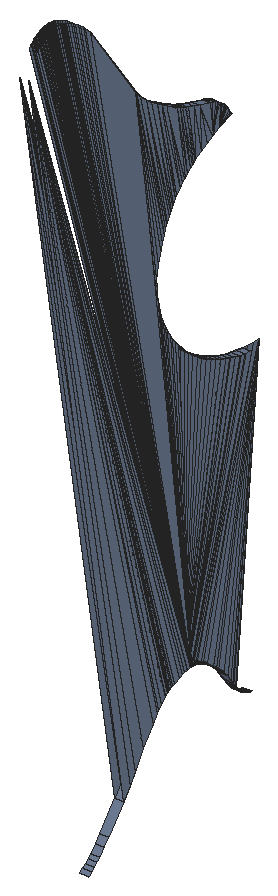
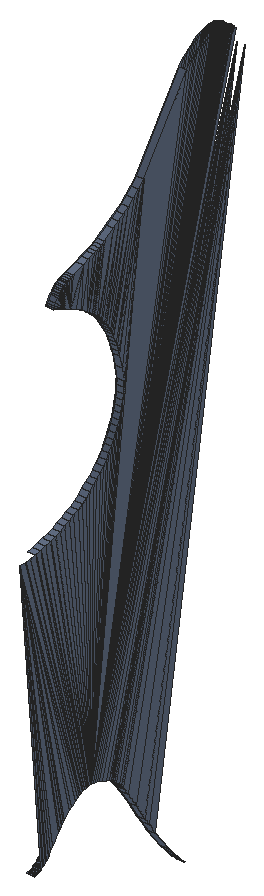
# SketchUp Ruby script. Lengths in inches.
U = 1.inch
M = Sketchup.active_model
def pt(a) = Geom::Point3d.new(a.map { |v| v * U })
def face(e, loops, mat)
  f = e.add_face(loops[0].map { |a| pt(a) })
  loops[1..].each { |l| e.add_face(l.map { |a| pt(a) }).erase! }
  f.material = f.back_material = mat if mat
  f
end
# faces: each face lists its corners as indices into pts; further lists are holes
def faces(e, pts, list, mat = nil) = list.each { |f| face(e, (f[0].is_a?(Array) ? f : [f]).map { |l| l.map { |i| pts[i] } }, mat) }
# xy, xz, yz: faces in a plane at the given z, y or x. An outline is a flat list of corners, or four numbers for a rectangle; further outlines are holes
def ring(l) = l.size == 4 ? [[l[0], l[1]], [l[2], l[1]], [l[2], l[3]], [l[0], l[3]]] : l.each_slice(2).to_a
def flat(e, list, mat, &to3) = list.each { |f| face(e, (f[0].is_a?(Array) ? f : [f]).map { |l| ring(l).map { |u, v| to3.(u, v) } }, mat) }
def xy(e, z, list, mat = nil) = flat(e, list, mat) { |x, y| [x, y, z] }
def xz(e, y, list, mat = nil) = flat(e, list, mat) { |x, z| [x, y, z] }
def yz(e, x, list, mat = nil) = flat(e, list, mat) { |y, z| [x, y, z] }
def lines(e, pts, list) = list.each { |a, b| e.add_line(pt(pts[a]), pt(pts[b])) }
# prism: a flat outline (further loops are holes) pulled along v
def prism(e, loops, v, mat = nil)
  f = face(e, loops, mat); d = Geom::Vector3d.new(v.map { |x| x * U })
  f.pushpull(f.normal.samedirection?(d) ? d.length : -d.length)
end
def box(e, o, s, mat = nil) = prism(e, [[o, [o[0] + s[0], o[1], o[2]], [o[0] + s[0], o[1] + s[1], o[2]], [o[0], o[1] + s[1], o[2]]]], [0, 0, s[2]], mat)
def at(x, y, z, deg = 0) = Geom::Transformation.translation(pt([x, y, z])) * Geom::Transformation.rotation(ORIGIN, Z_AXIS, deg.degrees)
def axes(o, x, y, z) = Geom::Transformation.new([*x, 0, *y, 0, *z, 0, *pt(o).to_a, 1])
def part(name) = M.definitions.add(name)
# library, detail: a bought-in or finely detailed component or shape, given as its bounding box
def library(name, o, s) = part(name).tap { |d| box(d.entities, o, s) }
def detail(e, o, s) = box(e.add_group.entities, o, s)
def put(e, d, t, mat = nil) = e.add_instance(d, t).tap { |i| i.material = mat if mat }
def group(e, t, mat = nil) = e.add_group.tap { |g| g.transformation = t; g.material = mat if mat }.entities
root = M.entities
M.materials.add("3D66_SU_1584934530605_002").color = [112, 126, 151]
xy(root,58.92,[[122.5,258.88,123.07,258.94]],"3D66_SU_1584934530605_002")
xy(root,58.93,[[122.5,258.6875,123.07,258.75],[122.5,258.75,123.07,258.8125]],"3D66_SU_1584934530605_002")
yz(root,122.5,[[252.91,53.28,244.87,100.53,253.42,53.97],[253.42,53.97,244.87,100.53,253.83,54.59],[253.83,54.59,244.87,100.53,254.58,55.75],[263.16,55.41,263.09,55.45,265.06,75.81],[263.09,55.45,263.01,55.5,265.06,75.81],
  [263.01,55.5,262.94,55.55,265.06,75.81],[262.94,55.55,262.87,55.61,265.06,75.81],[262.87,55.61,262.8,55.66,265.06,75.81],[262.8,55.66,262.73,55.73,265.06,75.81],[262.73,55.73,262.6,55.86,265.06,75.81],
  [254.58,55.75,244.87,100.53,255.36,56.85],[262.6,55.86,262.47,56,265.06,75.81],[262.47,56,262.35,56.15,265.06,75.81],[262.35,56.15,262.11,56.47,265.06,75.81],[262.11,56.47,261.65,57.11,265.06,75.81],
  [255.36,56.85,244.87,100.53,255.74,57.33],[261.65,57.11,261.53,57.26,265.06,75.81],[261.53,57.26,261.41,57.4,265.06,75.81],[255.74,57.33,244.87,100.53,255.92,57.55],[261.41,57.4,261.29,57.52,265.06,75.81],
  [261.29,57.52,261.23,57.58,265.06,75.81],[255.92,57.55,244.87,100.53,256.09,57.74],[261.23,57.58,261.17,57.64,265.06,75.81],[261.17,57.64,260.66,58.06,265.06,75.81],[256.09,57.74,244.87,100.53,256.38,58.03],
  [256.38,58.03,244.87,100.53,256.51,58.14],[260.66,58.06,260.4,58.25,265.06,75.81],[256.51,58.14,244.87,100.53,256.57,58.19],[256.57,58.19,244.87,100.53,256.63,58.24],[256.63,58.24,244.87,100.53,256.7,58.28],
  [260.4,58.25,260.14,58.42,265.06,75.81],[256.7,58.28,244.87,100.53,256.76,58.32],[256.76,58.32,244.87,100.53,256.83,58.36],[256.83,58.36,244.87,100.53,256.9,58.4],[256.9,58.4,244.87,100.53,257.05,58.47],
  [260.14,58.42,259.88,58.58,265.06,75.81],[257.05,58.47,244.87,100.53,257.23,58.54],[257.23,58.54,244.87,100.53,257.65,58.7],[259.88,58.58,259.76,58.65,265.06,75.81],[259.76,58.65,259.63,58.71,265.06,75.81],
  [257.65,58.7,244.87,100.53,257.88,58.77],[259.63,58.71,259.5,58.77,264.58,75.82],[259.63,58.71,264.58,75.82,265.06,75.81],[257.88,58.77,244.87,100.53,258.12,58.84],[259.5,58.77,259.375,58.8125,264.58,75.82],
  [259.375,58.8125,259.25,58.85,264.1,75.85],[259.375,58.8125,264.1,75.85,264.58,75.82],[258.12,58.84,244.87,100.53,258.25,58.87],[259.25,58.85,259.1875,58.87,263.63,75.9],[259.25,58.85,263.63,75.9,264.1,75.85],
  [258.25,58.87,244.87,100.53,258.37,58.89],[259.1875,58.87,259.125,58.89,263.63,75.9],[258.37,58.89,244.87,100.53,258.5,58.91],[259.125,58.89,259.07,58.9,263.17,75.97],[259.125,58.89,263.17,75.97,263.63,75.9],
  [259.07,58.9,259,58.91,263.17,75.97],[258.5,58.91,244.87,100.53,258.625,58.92],[259,58.91,258.94,58.92,262.72,76.05],[259,58.91,262.72,76.05,263.17,75.97],[258.625,58.92,245.66,101.97,245.79,102.11],
  [258.625,58.92,245.79,102.11,245.85,102.18],[258.625,58.92,245.85,102.18,245.92,102.24],[258.625,58.92,245.92,102.24,245.99,102.3],[258.625,58.92,245.99,102.3,246.06,102.36],[258.625,58.92,246.06,102.36,246.13,102.41],
  [258.625,58.92,246.13,102.41,246.2,102.46],[258.625,58.92,246.2,102.46,246.27,102.51],[258.625,58.92,246.27,102.51,246.35,102.55],[258.625,58.92,246.35,102.55,246.42,102.59],[258.625,58.92,246.42,102.59,246.5,102.625],
  [258.625,58.92,246.5,102.625,246.57,102.65],[258.625,58.92,246.57,102.65,246.65,102.68],[258.625,58.92,246.65,102.68,246.73,102.7],[258.625,58.92,246.73,102.7,246.81,102.72],[258.625,58.92,246.81,102.72,246.89,102.74],
  [258.625,58.92,246.89,102.74,246.97,102.75],[258.625,58.92,246.97,102.75,247.05,102.76],[258.625,58.92,247.05,102.76,247.13,102.77],[258.625,58.92,247.13,102.77,247.22,102.77],[258.625,58.92,247.22,102.77,247.31,102.77],
  [258.625,58.92,247.31,102.77,247.39,102.76],[258.625,58.92,247.39,102.76,247.48,102.75],[258.625,58.92,247.48,102.75,247.57,102.74],[258.625,58.92,247.57,102.74,247.66,102.72],[258.625,58.92,247.66,102.72,247.75,102.7],
  [258.625,58.92,247.75,102.7,247.85,102.68],[258.625,58.92,247.85,102.68,247.94,102.65],[258.625,58.92,247.94,102.65,248.04,102.62],[258.625,58.92,248.04,102.62,248.23,102.54],[258.625,58.92,248.23,102.54,248.43,102.46],
  [258.625,58.92,248.43,102.46,248.625,102.35],[258.625,58.92,248.625,102.35,248.83,102.23],[258.625,58.92,248.83,102.23,249.03,102.1],[258.625,58.92,249.03,102.1,249.24,101.95],[258.625,58.92,249.24,101.95,249.45,101.79],
  [258.625,58.92,249.45,101.79,249.67,101.61],[258.625,58.92,249.67,101.61,250.1,101.21],[258.625,58.92,250.1,101.21,253.92,95.88],[258.625,58.92,253.92,95.88,255.73,82.82],[258.625,58.92,255.73,82.82,255.79,82.43],
  [258.625,58.92,255.79,82.43,255.875,82.05],[258.625,58.92,255.875,82.05,255.98,81.67],[258.625,58.92,255.98,81.67,256.11,81.3],[258.625,58.92,256.11,81.3,256.25,80.9375],[258.625,58.92,256.25,80.9375,256.42,80.58],
  [258.625,58.92,256.42,80.58,256.61,80.24],[258.625,58.92,256.61,80.24,256.82,79.9],[258.625,58.92,256.82,79.9,257.04,79.57],[258.625,58.92,257.04,79.57,257.29,79.25],[258.625,58.92,257.29,79.25,257.55,78.95],
  [258.625,58.92,257.55,78.95,257.83,78.65],[258.625,58.92,257.83,78.65,258.12,78.37],[258.625,58.92,258.12,78.37,258.43,78.1],[258.625,58.92,258.43,78.1,258.76,77.84],[258.625,58.92,258.76,77.84,259.1,77.59],
  [258.625,58.92,259.1,77.59,259.45,77.36],[258.625,58.92,259.45,77.36,259.82,77.14],[258.625,58.92,259.82,77.14,260.2,76.94],[258.625,58.92,260.2,76.94,260.59,76.75],[258.625,58.92,260.59,76.75,261,76.58],
  [258.625,58.92,261,76.58,261.41,76.42],[258.625,58.92,261.41,76.42,261.84,76.28],[258.625,58.92,261.84,76.28,258.6875,58.93],[258.88,58.92,258.8125,58.93,262.27,76.16],[258.88,58.92,262.27,76.16,262.72,76.05],
  [258.88,58.92,262.72,76.05,258.94,58.92],[258.6875,58.93,261.84,76.28,258.75,58.93],[258.75,58.93,261.84,76.28,262.27,76.16],[258.75,58.93,262.27,76.16,258.8125,58.93],[255.73,82.82,253.92,95.88,255.7,83.22],
  [255.7,83.22,253.92,95.88,255.68,83.62],[255.68,83.62,253.92,95.88,255.85,84.54],[255.85,84.54,253.92,95.88,256.05,85.37],[256.05,85.37,253.92,95.88,256.17,85.75],[256.17,85.75,253.92,95.88,256.3,86.12],
  [256.3,86.12,253.92,95.88,254.38,95.42],[256.3,86.12,254.38,95.42,256.44,86.46],[256.44,86.46,254.38,95.42,256.59,86.79],[256.59,86.79,254.38,95.42,254.83,95.03],[256.59,86.79,254.83,95.03,256.75,87.1],
  [256.75,87.1,254.83,95.03,256.92,87.39],[256.92,87.39,254.83,95.03,255.28,94.68],[256.92,87.39,255.28,94.68,257.1,87.66],[257.1,87.66,255.28,94.68,255.72,94.38],[257.1,87.66,255.72,94.38,257.28,87.92],
  [257.28,87.92,255.72,94.38,256.16,94.11],[257.28,87.92,256.16,94.11,257.47,88.17],[257.47,88.17,256.16,94.11,257.67,88.4],[257.67,88.4,256.16,94.11,256.6,93.86],[257.67,88.4,256.6,93.86,257.875,88.62],
  [257.875,88.62,256.6,93.86,258.09,88.82],[258.09,88.82,256.6,93.86,257.47,93.4],[258.09,88.82,257.47,93.4,258.31,89.02],[258.31,89.02,257.47,93.4,257.7,93.29],[258.31,89.02,257.7,93.29,258.53,89.2],
  [258.53,89.2,257.7,93.29,257.93,93.19],[258.53,89.2,257.93,93.19,258.76,89.375],[258.76,89.375,257.93,93.19,258.16,93.09],[258.76,89.375,258.16,93.09,258.99,89.54],[258.99,89.54,258.16,93.09,258.4,93.01],
  [258.99,89.54,258.4,93.01,258.88,92.86],[258.99,89.54,258.88,92.86,259.48,89.84],[259.48,89.84,258.88,92.86,259.35,92.72],[259.48,89.84,259.35,92.72,259.97,90.11],[259.97,90.11,259.35,92.72,260.48,90.36],
  [260.48,90.36,259.35,92.72,260.23,92.47],[260.48,90.36,260.23,92.47,260.43,92.41],[260.48,90.36,260.43,92.41,260.61,92.35],[260.48,90.36,260.61,92.35,260.78,92.28],[260.48,90.36,260.78,92.28,260.86,92.24],
  [260.48,90.36,260.86,92.24,260.93,92.21],[260.48,90.36,260.93,92.21,261.0625,92.13],[260.48,90.36,261.0625,92.13,261,90.59],[261,90.59,261.0625,92.13,261.18,92.06],[261,90.59,261.18,92.06,261.28,91.98],
  [261,90.59,261.28,91.98,261.375,91.91],[261,90.59,261.375,91.91,261.45,91.84],[261,90.59,261.45,91.84,261.52,91.76],[261,90.59,261.52,91.76,261.58,91.6875],[261,90.59,261.58,91.6875,261.64,91.61],
  [261,90.59,261.64,91.61,261.83,91.32],[261,90.59,261.83,91.32,261.93,91.17],[261,90.59,261.93,91.17,261.99,91.09],[261,90.59,261.99,91.09,262.06,91.02]],"3D66_SU_1584934530605_002")
yz(root,123.07,[[252.91,53.28,253.42,53.97,244.87,100.53],[253.42,53.97,253.83,54.59,244.87,100.53],[253.83,54.59,254.58,55.75,244.87,100.53],[254.58,55.75,255.36,56.85,244.87,100.53],[255.36,56.85,255.74,57.33,244.87,100.53],
  [255.74,57.33,255.92,57.55,244.87,100.53],[255.92,57.55,256.09,57.74,244.87,100.53],[256.09,57.74,256.38,58.03,244.87,100.53],[256.38,58.03,256.51,58.14,244.87,100.53],[256.51,58.14,256.57,58.19,244.87,100.53],
  [256.57,58.19,256.63,58.24,244.87,100.53],[256.63,58.24,256.7,58.28,244.87,100.53],[256.7,58.28,256.76,58.32,244.87,100.53],[256.76,58.32,256.83,58.36,244.87,100.53],[256.83,58.36,256.9,58.4,244.87,100.53],
  [256.9,58.4,257.05,58.47,244.87,100.53],[257.05,58.47,257.23,58.54,244.87,100.53],[257.23,58.54,257.65,58.7,244.87,100.53],[257.65,58.7,257.88,58.77,244.87,100.53],[257.88,58.77,258.12,58.84,244.87,100.53],
  [258.12,58.84,258.25,58.87,244.87,100.53],[258.25,58.87,258.37,58.89,244.87,100.53],[258.37,58.89,258.5,58.91,244.87,100.53],[258.5,58.91,258.625,58.92,244.87,100.53],[258.625,58.92,245.66,101.97,245.53,101.81],
  [258.625,58.92,245.79,102.11,245.66,101.97],[258.625,58.92,245.85,102.18,245.79,102.11],[258.625,58.92,245.92,102.24,245.85,102.18],[258.625,58.92,245.99,102.3,245.92,102.24],[258.625,58.92,246.06,102.36,245.99,102.3],
  [258.625,58.92,246.13,102.41,246.06,102.36],[258.625,58.92,246.2,102.46,246.13,102.41],[258.625,58.92,246.27,102.51,246.2,102.46],[258.625,58.92,246.35,102.55,246.27,102.51],[258.625,58.92,246.42,102.59,246.35,102.55],
  [258.625,58.92,246.5,102.625,246.42,102.59],[258.625,58.92,246.57,102.65,246.5,102.625],[258.625,58.92,246.65,102.68,246.57,102.65],[258.625,58.92,246.73,102.7,246.65,102.68],[258.625,58.92,246.81,102.72,246.73,102.7],
  [258.625,58.92,246.89,102.74,246.81,102.72],[258.625,58.92,246.97,102.75,246.89,102.74],[258.625,58.92,247.05,102.76,246.97,102.75],[258.625,58.92,247.13,102.77,247.05,102.76],[258.625,58.92,247.22,102.77,247.13,102.77],
  [258.625,58.92,247.31,102.77,247.22,102.77],[258.625,58.92,247.39,102.76,247.31,102.77],[258.625,58.92,247.48,102.75,247.39,102.76],[258.625,58.92,247.57,102.74,247.48,102.75],[258.625,58.92,247.66,102.72,247.57,102.74],
  [258.625,58.92,247.75,102.7,247.66,102.72],[258.625,58.92,247.85,102.68,247.75,102.7],[258.625,58.92,247.94,102.65,247.85,102.68],[258.625,58.92,248.04,102.62,247.94,102.65],[258.625,58.92,248.23,102.54,248.04,102.62],
  [258.625,58.92,248.43,102.46,248.23,102.54],[258.625,58.92,248.625,102.35,248.43,102.46],[258.625,58.92,248.83,102.23,248.625,102.35],[258.625,58.92,249.03,102.1,248.83,102.23],[258.625,58.92,249.24,101.95,249.03,102.1],
  [258.625,58.92,249.45,101.79,249.24,101.95],[258.625,58.92,249.67,101.61,249.45,101.79],[258.625,58.92,250.1,101.21,249.67,101.61],[258.625,58.92,253.92,95.88,250.1,101.21],[258.625,58.92,255.73,82.82,253.92,95.88],
  [258.625,58.92,255.79,82.43,255.73,82.82],[258.625,58.92,255.875,82.05,255.79,82.43],[258.625,58.92,255.98,81.67,255.875,82.05],[258.625,58.92,256.11,81.3,255.98,81.67],[258.625,58.92,256.25,80.9375,256.11,81.3],
  [258.625,58.92,256.42,80.58,256.25,80.9375],[258.625,58.92,256.61,80.24,256.42,80.58],[258.625,58.92,256.82,79.9,256.61,80.24],[258.625,58.92,257.04,79.57,256.82,79.9],[258.625,58.92,257.29,79.25,257.04,79.57],
  [258.625,58.92,257.55,78.95,257.29,79.25],[255.73,82.82,255.7,83.22,253.92,95.88],[255.7,83.22,255.68,83.62,253.92,95.88],[255.68,83.62,255.85,84.54,253.92,95.88],[255.85,84.54,256.05,85.37,253.92,95.88],
  [256.05,85.37,256.17,85.75,253.92,95.88],[256.17,85.75,256.3,86.12,253.92,95.88],[256.3,86.12,254.38,95.42,253.92,95.88],[256.3,86.12,256.44,86.46,254.38,95.42],[256.44,86.46,256.59,86.79,254.38,95.42],
  [256.59,86.79,254.83,95.03,254.38,95.42],[256.59,86.79,256.75,87.1,254.83,95.03],[256.75,87.1,256.92,87.39,254.83,95.03],[256.92,87.39,255.28,94.68,254.83,95.03],[256.92,87.39,257.1,87.66,255.28,94.68],
  [257.1,87.66,255.72,94.38,255.28,94.68],[257.1,87.66,257.28,87.92,255.72,94.38],[257.28,87.92,256.16,94.11,255.72,94.38],[257.28,87.92,257.47,88.17,256.16,94.11],[257.47,88.17,257.67,88.4,256.16,94.11],
  [257.67,88.4,256.6,93.86,256.16,94.11],[257.67,88.4,257.875,88.62,256.6,93.86],[257.875,88.62,258.09,88.82,256.6,93.86],[258.09,88.82,257.47,93.4,256.6,93.86],[258.09,88.82,258.31,89.02,257.47,93.4],
  [258.31,89.02,257.7,93.29,257.47,93.4],[258.31,89.02,258.53,89.2,257.7,93.29],[258.53,89.2,257.93,93.19,257.7,93.29],[258.53,89.2,258.76,89.375,257.93,93.19],[258.76,89.375,258.16,93.09,257.93,93.19],
  [258.76,89.375,258.99,89.54,258.16,93.09],[258.99,89.54,258.4,93.01,258.16,93.09],[258.99,89.54,258.88,92.86,258.4,93.01],[258.99,89.54,259.48,89.84,258.88,92.86],[259.48,89.84,259.35,92.72,258.88,92.86],
  [259.48,89.84,259.97,90.11,259.35,92.72],[259.97,90.11,260.48,90.36,259.35,92.72],[260.48,90.36,260.23,92.47,259.35,92.72],[260.48,90.36,260.43,92.41,260.23,92.47],[260.48,90.36,260.61,92.35,260.43,92.41],
  [260.48,90.36,260.78,92.28,260.61,92.35],[260.48,90.36,260.86,92.24,260.78,92.28],[260.48,90.36,260.93,92.21,260.86,92.24],[260.48,90.36,261,90.59,261.0625,92.13],[260.48,90.36,261.0625,92.13,260.93,92.21],
  [261,90.59,261.18,92.06,261.0625,92.13],[261,90.59,261.28,91.98,261.18,92.06],[261,90.59,261.375,91.91,261.28,91.98],[261,90.59,261.45,91.84,261.375,91.91],[261,90.59,261.52,91.76,261.45,91.84],
  [261,90.59,261.58,91.6875,261.52,91.76],[261,90.59,261.64,91.61,261.58,91.6875],[261,90.59,261.83,91.32,261.64,91.61],[261,90.59,261.93,91.17,261.83,91.32],[261,90.59,261.99,91.09,261.93,91.17],
  [261,90.59,262.06,91.02,261.99,91.09]],"3D66_SU_1584934530605_002")
p = [[123.07,249.96,50.03],[122.5,249.96,50.03],[122.5,250.21,50.21],[123.07,250.21,50.21],[122.5,250.44,50.4],[123.07,250.44,50.4],
  [122.5,250.66,50.6],[123.07,250.66,50.6],[122.5,250.88,50.81],[123.07,250.88,50.81],[122.5,251.28,51.23],[123.07,251.28,51.23],
  [122.5,251.65,51.66],[123.07,251.65,51.66],[122.5,252.91,53.28],[123.07,252.91,53.28],[122.5,253.42,53.97],[123.07,253.42,53.97],
  [122.5,253.83,54.59],[123.07,253.83,54.59],[122.5,254.58,55.75],[123.07,254.58,55.75],[123.07,263.58,55.26],[122.5,263.58,55.26],
  [122.5,263.67,55.24],[123.07,263.67,55.24],[122.5,263.76,55.22],[123.07,263.76,55.22],[123.07,263.24,55.37],[122.5,263.24,55.37],
  [122.5,263.32,55.34],[123.07,263.32,55.34],[122.5,263.41,55.31],[123.07,263.41,55.31],[122.5,263.49,55.28],[123.07,263.49,55.28],
  [123.07,263.09,55.45],[122.5,263.09,55.45],[122.5,263.16,55.41],[123.07,263.16,55.41],[122.5,262.94,55.55],[123.07,263.01,55.5],
  [123.07,262.94,55.55],[122.5,263.01,55.5],[122.5,262.8,55.66],[123.07,262.87,55.61],[123.07,262.8,55.66],[122.5,262.87,55.61],
  [122.5,255.36,56.85],[123.07,255.36,56.85],[123.07,262.6,55.86],[122.5,262.6,55.86],[122.5,262.73,55.73],[123.07,262.73,55.73],
  [123.07,262.47,56],[122.5,262.47,56],[123.07,262.35,56.15],[122.5,262.35,56.15],[123.07,262.11,56.47],[122.5,262.11,56.47],
  [123.07,261.65,57.11],[122.5,261.65,57.11],[122.5,255.74,57.33],[123.07,255.74,57.33],[123.07,261.53,57.26],[122.5,261.53,57.26],
  [122.5,255.92,57.55],[123.07,255.92,57.55],[123.07,261.41,57.4],[122.5,261.41,57.4],[123.07,261.29,57.52],[122.5,261.29,57.52],
  [122.5,256.09,57.74],[123.07,256.09,57.74],[122.5,261.23,57.58],[123.07,261.23,57.58],[123.07,260.66,58.06],[122.5,260.66,58.06],
  [122.5,261.17,57.64],[123.07,261.17,57.64],[122.5,256.38,58.03],[123.07,256.38,58.03],[122.5,256.51,58.14],[123.07,256.51,58.14],
  [123.07,256.57,58.19],[122.5,256.57,58.19],[123.07,260.4,58.25],[122.5,260.4,58.25],[123.07,256.63,58.24],[122.5,256.63,58.24],
  [123.07,256.7,58.28],[122.5,256.7,58.28],[123.07,260.14,58.42],[122.5,260.14,58.42],[123.07,256.76,58.32],[122.5,256.76,58.32],
  [123.07,256.83,58.36],[122.5,256.83,58.36],[122.5,256.9,58.4],[123.07,256.9,58.4],[122.5,257.05,58.47],[123.07,257.05,58.47],
  [123.07,259.88,58.58],[122.5,259.88,58.58],[122.5,257.23,58.54],[123.07,257.23,58.54],[122.5,257.65,58.7],[123.07,257.65,58.7],
  [123.07,259.63,58.71],[122.5,259.63,58.71],[122.5,259.76,58.65],[123.07,259.76,58.65],[122.5,257.88,58.77],[123.07,257.88,58.77],
  [123.07,259.5,58.77],[122.5,259.5,58.77],[122.5,258.12,58.84],[123.07,258.12,58.84],[122.5,258.25,58.87],[123.07,258.25,58.87],
  [123.07,259.25,58.85],[122.5,259.25,58.85],[122.5,259.375,58.8125],[123.07,259.375,58.8125],[122.5,258.37,58.89],[123.07,258.37,58.89],
  [122.5,258.5,58.91],[123.07,258.5,58.91],[122.5,258.625,58.92],[123.07,258.625,58.92],[122.5,258.6875,58.93],[123.07,258.6875,58.93],
  [123.07,258.8125,58.93],[122.5,258.8125,58.93],[122.5,258.88,58.92],[123.07,258.88,58.92],[123.07,258.94,58.92],[122.5,258.94,58.92],
  [122.5,259,58.91],[123.07,259,58.91],[122.5,259.07,58.9],[123.07,259.07,58.9],[122.5,259.125,58.89],[123.07,259.125,58.89],
  [122.5,259.1875,58.87],[123.07,259.1875,58.87],[123.07,263.63,75.9],[122.5,263.63,75.9],[122.5,263.17,75.97],[123.07,263.17,75.97],
  [122.5,262.72,76.05],[123.07,262.72,76.05],[122.5,262.27,76.16],[123.07,262.27,76.16],[122.5,261.84,76.28],[123.07,261.84,76.28],
  [122.5,261.41,76.42],[123.07,261.41,76.42],[122.5,261,76.58],[123.07,261,76.58],[122.5,260.59,76.75],[123.07,260.59,76.75],
  [122.5,260.2,76.94],[123.07,260.2,76.94],[122.5,259.82,77.14],[123.07,259.82,77.14],[122.5,259.45,77.36],[123.07,259.45,77.36],
  [122.5,259.1,77.59],[123.07,259.1,77.59],[122.5,258.76,77.84],[123.07,258.76,77.84],[122.5,258.43,78.1],[123.07,258.43,78.1],
  [122.5,258.12,78.37],[123.07,258.12,78.37],[122.5,257.83,78.65],[123.07,257.83,78.65],[122.5,257.55,78.95],[123.07,257.55,78.95],
  [122.5,257.29,79.25],[123.07,257.29,79.25],[122.5,257.04,79.57],[123.07,257.04,79.57],[122.5,256.82,79.9],[123.07,256.82,79.9],
  [122.5,256.61,80.24],[123.07,256.61,80.24],[122.5,256.42,80.58],[123.07,256.42,80.58],[122.5,256.25,80.9375],[123.07,256.25,80.9375],
  [122.5,256.11,81.3],[123.07,256.11,81.3],[122.5,255.98,81.67],[123.07,255.98,81.67],[122.5,255.875,82.05],[123.07,255.875,82.05],
  [122.5,255.79,82.43],[123.07,255.79,82.43],[122.5,255.73,82.82],[123.07,255.73,82.82],[122.5,255.7,83.22],[123.07,255.7,83.22],
  [122.5,255.68,83.62],[123.07,255.68,83.62],[122.5,255.85,84.54],[123.07,255.85,84.54],[122.5,256.05,85.37],[123.07,256.05,85.37],
  [122.5,256.17,85.75],[123.07,256.17,85.75],[122.5,256.3,86.12],[123.07,256.3,86.12],[122.5,256.44,86.46],[123.07,256.44,86.46],
  [122.5,256.59,86.79],[123.07,256.59,86.79],[122.5,256.75,87.1],[123.07,256.75,87.1],[122.5,256.92,87.39],[123.07,256.92,87.39],
  [122.5,257.1,87.66],[123.07,257.1,87.66],[122.5,257.28,87.92],[123.07,257.28,87.92],[122.5,257.47,88.17],[123.07,257.47,88.17],
  [122.5,257.67,88.4],[123.07,257.67,88.4],[122.5,257.875,88.62],[123.07,257.875,88.62],[122.5,258.09,88.82],[123.07,258.09,88.82],
  [122.5,258.31,89.02],[123.07,258.31,89.02],[122.5,258.53,89.2],[123.07,258.53,89.2],[122.5,258.76,89.375],[123.07,258.76,89.375],
  [122.5,258.99,89.54],[123.07,258.99,89.54],[122.5,259.48,89.84],[123.07,259.48,89.84],[122.5,259.97,90.11],[123.07,259.97,90.11],
  [122.5,260.48,90.36],[123.07,260.48,90.36],[122.5,261,90.59],[123.07,261,90.59],[122.5,262.06,91.02],[123.07,262.06,91.02],
  [122.5,261.99,91.09],[123.07,261.99,91.09],[122.5,261.93,91.17],[123.07,261.93,91.17],[122.5,261.83,91.32],[123.07,261.83,91.32],
  [122.5,261.64,91.61],[123.07,261.64,91.61],[122.5,261.58,91.6875],[123.07,261.58,91.6875],[122.5,261.52,91.76],[123.07,261.52,91.76],
  [123.07,261.45,91.84],[122.5,261.45,91.84],[122.5,261.375,91.91],[123.07,261.375,91.91],[122.5,261.28,91.98],[123.07,261.28,91.98],
  [122.5,261.18,92.06],[123.07,261.18,92.06],[123.07,261.0625,92.13],[122.5,261.0625,92.13],[122.5,260.93,92.21],[123.07,260.93,92.21],
  [123.07,260.86,92.24],[122.5,260.86,92.24],[122.5,260.78,92.28],[123.07,260.78,92.28],[123.07,260.61,92.35],[122.5,260.61,92.35],
  [122.5,260.43,92.41],[123.07,260.43,92.41],[122.5,260.23,92.47],[123.07,260.23,92.47],[122.5,259.35,92.72],[123.07,259.35,92.72],
  [122.5,258.88,92.86],[123.07,258.88,92.86],[122.5,258.4,93.01],[123.07,258.4,93.01],[122.5,258.16,93.09],[123.07,258.16,93.09],
  [122.5,257.93,93.19],[123.07,257.93,93.19],[122.5,257.7,93.29],[123.07,257.7,93.29],[122.5,257.47,93.4],[123.07,257.47,93.4],
  [122.5,256.6,93.86],[123.07,256.6,93.86],[122.5,256.16,94.11],[123.07,256.16,94.11],[122.5,255.72,94.38],[123.07,255.72,94.38],
  [122.5,255.28,94.68],[123.07,255.28,94.68],[122.5,254.83,95.03],[123.07,254.83,95.03],[122.5,254.38,95.42],[123.07,254.38,95.42],
  [122.5,253.92,95.88],[123.07,253.92,95.88],[122.5,250.1,101.21],[123.07,250.1,101.21]]
faces(root,p,[[0,1,2,3],[3,2,4,5],[5,4,6,7],[7,6,8,9],[9,8,10,11],[11,10,12,13],[13,12,14,15],[15,14,16,17],
  [17,16,18,19],[19,18,20,21],[22,23,24,25],[25,24,26,27],[28,29,30,31],[31,30,32,33],[33,32,34,35],[35,34,23,22],
  [36,37,38,39],[39,38,29,28],[40,41,42],[40,43,41],[43,36,41],[43,37,36],[44,45,46],[44,47,45],
  [47,42,45],[47,40,42],[21,20,48,49],[50,51,52,53],[52,46,53],[52,44,46],[54,55,51,50],[56,57,55,54],
  [58,59,57,56],[60,61,59,58],[49,48,62,63],[64,65,61,60],[63,62,66,67],[68,69,65,64],[70,71,69,68],[67,66,72,73],
  [74,70,75],[74,71,70],[76,77,78,79],[78,75,79],[78,74,75],[73,72,80,81],[81,80,82,83],[82,84,83],
  [82,85,84],[86,87,77,76],[85,88,84],[85,89,88],[89,90,88],[89,91,90],[92,93,87,86],[91,94,90],
  [91,95,94],[95,96,94],[95,97,96],[96,97,98,99],[99,98,100,101],[102,103,93,92],[101,100,104,105],[105,104,106,107],
  [108,109,110,111],[111,110,103,102],[107,106,112,113],[114,115,109,108],[113,112,116,117],[117,116,118,119],[120,121,122,123],[123,122,115,114],
  [119,118,124,125],[125,124,126,127],[127,126,128,129],[129,128,130,131],[132,133,134,135],[136,137,138,139],[139,138,140,141],[141,140,142,143],
  [143,142,144,145],[145,144,121,120],[146,147,148,149],[149,148,150,151],[151,150,152,153],[153,152,154,155],[155,154,156,157],[157,156,158,159],
  [159,158,160,161],[161,160,162,163],[163,162,164,165],[165,164,166,167],[167,166,168,169],[169,168,170,171],[171,170,172,173],[173,172,174,175],
  [175,174,176,177],[177,176,178,179],[179,178,180,181],[181,180,182,183],[183,182,184,185],[185,184,186,187],[187,186,188,189],[189,188,190,191],
  [191,190,192,193],[193,192,194,195],[195,194,196,197],[197,196,198,199],[199,198,200,201],[201,200,202,203],[203,202,204,205],[205,204,206,207],
  [207,206,208,209],[209,208,210,211],[211,210,212,213],[213,212,214,215],[215,214,216,217],[217,216,218,219],[219,218,220,221],[221,220,222,223],
  [223,222,224,225],[225,224,226,227],[227,226,228,229],[229,228,230,231],[231,230,232,233],[233,232,234,235],[235,234,236,237],[237,236,238,239],
  [239,238,240,241],[241,240,242,243],[243,242,244,245],[245,244,246,247],[247,246,248,249],[249,248,250,251],[251,250,252,253],[253,252,254,255],
  [255,254,256,257],[257,256,258,259],[259,258,260,261],[261,260,262,263],[264,265,266,267],[262,265,264],[262,264,263],[267,266,268,269],
  [269,268,270,271],[272,273,274,275],[271,270,273,272],[276,277,278,279],[275,274,277,276],[280,281,282,283],[279,278,281,280],[283,282,284,285],
  [285,284,286,287],[287,286,288,289],[289,288,290,291],[291,290,292,293],[293,292,294,295],[295,294,296,297],[297,296,298,299],[299,298,300,301],
  [301,300,302,303],[303,302,304,305],[305,304,306,307],[307,306,308,309],[309,308,310,311],[311,310,312,313],[313,312,314,315]],"3D66_SU_1584934530605_002")
